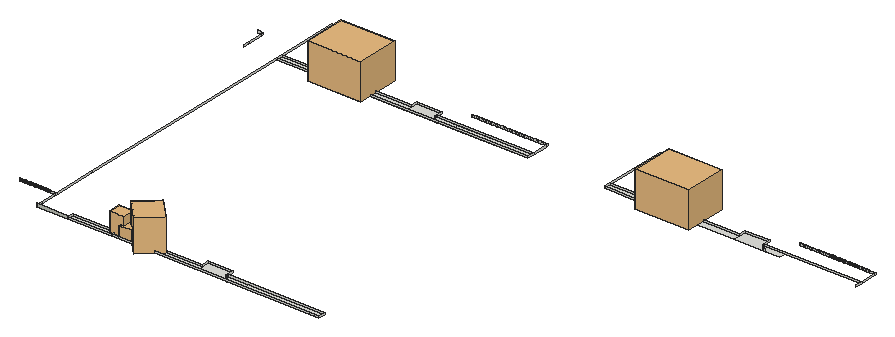
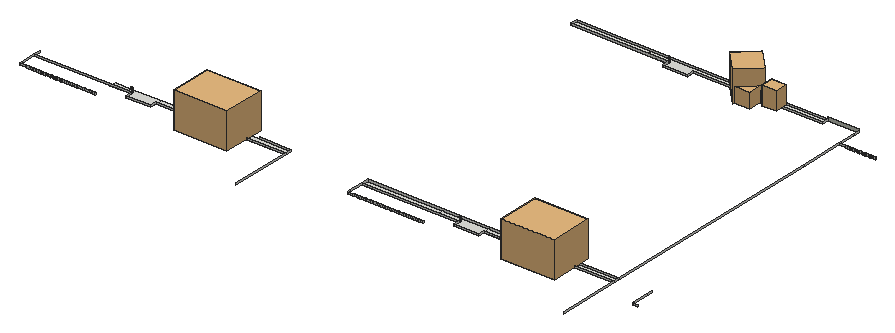
# SketchUp Ruby script. Lengths in inches.
U = 1.inch
M = Sketchup.active_model
def pt(a) = Geom::Point3d.new(a.map { |v| v * U })
def face(e, loops, mat)
  f = e.add_face(loops[0].map { |a| pt(a) })
  loops[1..].each { |l| e.add_face(l.map { |a| pt(a) }).erase! }
  f.material = f.back_material = mat if mat
  f
end
# faces: each face lists its corners as indices into pts; further lists are holes
def faces(e, pts, list, mat = nil) = list.each { |f| face(e, (f[0].is_a?(Array) ? f : [f]).map { |l| l.map { |i| pts[i] } }, mat) }
# xy, xz, yz: faces in a plane at the given z, y or x. An outline is a flat list of corners, or four numbers for a rectangle; further outlines are holes
def ring(l) = l.size == 4 ? [[l[0], l[1]], [l[2], l[1]], [l[2], l[3]], [l[0], l[3]]] : l.each_slice(2).to_a
def flat(e, list, mat, &to3) = list.each { |f| face(e, (f[0].is_a?(Array) ? f : [f]).map { |l| ring(l).map { |u, v| to3.(u, v) } }, mat) }
def xy(e, z, list, mat = nil) = flat(e, list, mat) { |x, y| [x, y, z] }
def xz(e, y, list, mat = nil) = flat(e, list, mat) { |x, z| [x, y, z] }
def yz(e, x, list, mat = nil) = flat(e, list, mat) { |y, z| [x, y, z] }
def lines(e, pts, list) = list.each { |a, b| e.add_line(pt(pts[a]), pt(pts[b])) }
# prism: a flat outline (further loops are holes) pulled along v
def prism(e, loops, v, mat = nil)
  f = face(e, loops, mat); d = Geom::Vector3d.new(v.map { |x| x * U })
  f.pushpull(f.normal.samedirection?(d) ? d.length : -d.length)
end
def box(e, o, s, mat = nil) = prism(e, [[o, [o[0] + s[0], o[1], o[2]], [o[0] + s[0], o[1] + s[1], o[2]], [o[0], o[1] + s[1], o[2]]]], [0, 0, s[2]], mat)
def at(x, y, z, deg = 0) = Geom::Transformation.translation(pt([x, y, z])) * Geom::Transformation.rotation(ORIGIN, Z_AXIS, deg.degrees)
def axes(o, x, y, z) = Geom::Transformation.new([*x, 0, *y, 0, *z, 0, *pt(o).to_a, 1])
def part(name) = M.definitions.add(name)
# library, detail: a bought-in or finely detailed component or shape, given as its bounding box
def library(name, o, s) = part(name).tap { |d| box(d.entities, o, s) }
def detail(e, o, s) = box(e.add_group.entities, o, s)
def put(e, d, t, mat = nil) = e.add_instance(d, t).tap { |i| i.material = mat if mat }
def group(e, t, mat = nil) = e.add_group.tap { |g| g.transformation = t; g.material = mat if mat }.entities
root = M.entities
M.materials.add("Material__1").color = [95, 70, 46]
M.materials.add("[Pavers with Grass Herringbone]").color = [197, 201, 190]
M.materials.add("wire_5").color = [232, 232, 232]
c1 = library("Sem+nome (1)",[20.77,3.52,-2.22],[96.42,122.82,82.56])
c2 = library("Agrupar\#178",[0,0,0],[37.88,32.09,49.42])
c3 = library("Agrupar\#177",[0,0,0],[36.52,33.08,30.88])
c4 = library("Agrupar\#154",[0,0,0],[41.26,44.6,38.97])
c5 = library("Palm",[82.2,-9.29,-2.36],[51.18,55.77,65.42])
c6 = library("Pinch Pot",[-27.95,-27.95,0],[55.9,55.9,47.42])
c7 = library("Group\#386",[-915.9375,-34.5,735.6],[41.04,40.85,6.81])
c8 = library("Group\#403",[-912.1,-32.49,735.82],[33.14,36.63,9.55])
c9 = part("Potted palm")
put(c9.entities,c5,axes([3796.42,-10488.37,43.97],[0,116.51338,0],[-116.51338,0,0],[0,0,116.51338]))
put(c9.entities,c6,axes([1647.67,1801.1875,0],[0,30.58476,0],[-30.58476,0,0],[0,0,45.1095]))
put(c9.entities,c7,axes([32580.48,2279.8125,-23417.78],[34.48768,0,0],[0,34.48768,0],[0,0,34.48768]),"Material__1")
put(c9.entities,c8,axes([32580.48,2279.8125,-23417.78],[34.48768,0,0],[0,34.48768,0],[0,0,34.48768]),"wire_5")
xy(root,-12.3125,[[1134.71,147.25,1235.9,162.52],[1300.19,147.25,1302.19,147.38,1304.14,147.77,1306.03,148.41,1307.83,149.3,1309.49,150.4,1310.99,151.72,1312.3,153.22,1313.41,154.88,1314.3,156.67,1314.9375,158.57,1315.33,160.52,1315.46,162.52,1432.9,162.52,1432.9,147.25],[1432.9,147.25,1432.9,178.0625,1489.92,178.0625,1489.92,162.33,1490.05,160.36,1490.43,158.43,1491.07,156.56,1491.9375,154.79,1493.03,153.15,1494.34,151.67,1495.82,150.37,1497.46,149.27,1499.23,148.4,1501.1,147.76,1503.03,147.38,1505,147.25],[1505,147.25,1503.03,147.38,1501.1,147.76,1499.23,148.4,1497.46,149.27,1495.82,150.37,1494.34,151.67,1493.03,153.15,1491.9375,154.79,1491.07,156.56,1490.43,158.43,1490.05,160.36,1489.92,162.33,1539,162.33,1539,147.25],[1539,147.25,1713.52,162.33],
  [1063.02,838.14,1164.21,853.41],[1228.5,838.14,1230.5,838.27,1232.46,838.66,1234.35,839.31,1236.14,840.19,1237.8,841.3,1239.3,842.62,1240.62,844.12,1241.73,845.78,1242.61,847.57,1243.25,849.46,1243.64,851.42,1243.77,853.41,1361.21,853.41,1361.21,838.14],[1361.21,838.14,1361.21,868.96,1418.23,868.96,1418.23,853.22,1418.36,851.26,1418.74,849.32,1419.38,847.45,1420.25,845.68,1421.35,844.04,1422.65,842.5625,1424.13,841.26,1425.77,840.16,1427.54,839.29,1429.41,838.66,1431.34,838.27,1433.3125,838.14],[1433.3125,838.14,1431.34,838.27,1429.41,838.66,1427.54,839.29,1425.77,840.16,1424.13,841.26,1422.65,842.5625,1421.35,844.04,1420.25,845.68,1419.38,847.45,1418.74,849.32,1418.36,851.26,1418.23,853.22,1467.3125,853.22,1467.3125,838.14],[1467.3125,838.14,1641.83,853.22],
  [1817.65,838.14,1918.83,853.41],[1983.13,838.14,1985.12,838.27,1987.08,838.66,1988.97,839.31,1990.76,840.19,1992.42,841.3,1993.93,842.62,1995.24,844.12,1996.35,845.78,1997.23,847.57,1997.875,849.46,1998.27,851.42,1998.4,853.41,2115.83,853.41,2115.83,838.14],[2115.83,838.14,2115.83,868.96,2172.86,868.96,2172.86,853.22,2172.98,851.26,2173.37,849.32,2174,847.45,2174.875,845.68,2175.97,844.04,2177.27,842.5625,2178.76,841.26,2180.4,840.16,2182.17,839.29,2184.03,838.66,2185.97,838.27,2187.9375,838.14],[2187.9375,838.14,2185.97,838.27,2184.03,838.66,2182.17,839.29,2180.4,840.16,2178.76,841.26,2177.27,842.5625,2175.97,844.04,2174.875,845.68,2174,847.45,2173.37,849.32,2172.98,851.26,2172.86,853.22,2221.9375,853.22,2221.9375,838.14]])
xz(root,147.25,[[1134.71,-12.3125,1235.9,-8],[1235.9,-12.3125,1300.19,-8],[1300.19,-12.3125,1713.52,-8]])
xz(root,147.25,[[1063.02,-12.3125,1134.71,-4.67]],"[Pavers with Grass Herringbone]")
xz(root,162.33,[[1489.92,-12.3125,1713.52,-8]])
xz(root,162.52,[[1134.71,-12.3125,1235.9,-8],[1235.9,-12.3125,1315.46,-8],[1315.46,-12.3125,1432.9,-8]])
xz(root,178.0625,[[1432.9,-12.3125,1489.92,-8]])
xz(root,203.875,[[978.875,-12.3125,982.125,-8],[982.875,-12.3125,986.125,-8],[986.875,-12.3125,990.125,-8],[990.875,-12.3125,994.125,-8],[994.875,-12.3125,998.125,-8],
  [998.875,-12.3125,1002.125,-8],[1002.875,-12.3125,1006.125,-8],[1006.875,-12.3125,1010.125,-8],[1010.875,-12.3125,1014.125,-8],[1014.875,-12.3125,1018.125,-8],
  [1018.875,-12.3125,1022.125,-8],[1022.875,-12.3125,1026.125,-8],[1026.875,-12.3125,1030.125,-8],[1030.875,-12.3125,1034.125,-8],[1034.875,-12.3125,1038.125,-8],
  [1038.875,-12.3125,1042.125,-8],[1042.875,-12.3125,1046.125,-8],[1046.875,-12.3125,1050.125,-8],[1050.125,-12.3125,1063.02,-8]])
xz(root,204.875,[[978.125,-12.3125,978.875,-8],[982.125,-12.3125,982.875,-8],[986.125,-12.3125,986.875,-8],[990.125,-12.3125,990.875,-8],[994.125,-12.3125,994.875,-8],
  [998.125,-12.3125,998.875,-8],[1002.125,-12.3125,1002.875,-8],[1006.125,-12.3125,1006.875,-8],[1010.125,-12.3125,1010.875,-8],[1014.125,-12.3125,1014.875,-8],
  [1018.125,-12.3125,1018.875,-8],[1022.125,-12.3125,1022.875,-8],[1026.125,-12.3125,1026.875,-8],[1030.125,-12.3125,1030.875,-8],[1034.125,-12.3125,1034.875,-8],
  [1038.125,-12.3125,1038.875,-8],[1042.125,-12.3125,1042.875,-8],[1046.125,-12.3125,1046.875,-8]])
xz(root,838.14,[[1063.02,-12.3125,1134.71,-8],[1134.71,-12.3125,1164.21,-8],[1164.21,-12.3125,1228.5,-8],[1228.5,-12.3125,1641.83,-8],[1817.65,-12.3125,1889.33,-8],
  [1918.83,-12.3125,1983.13,-8]])
xz(root,853.22,[[1418.23,-12.3125,1641.83,-8],[2172.86,-12.3125,2396.46,-8]])
xz(root,853.41,[[1063.02,-12.3125,1164.21,-8],[1164.21,-12.3125,1243.77,-8],[1243.77,-12.3125,1361.21,-8],[1817.65,-12.3125,1918.83,-8],[1918.83,-12.3125,1998.4,-8],
  [1998.4,-12.3125,2115.83,-8]])
xz(root,868.96,[[1361.21,-12.3125,1418.23,-8],[2115.83,-12.3125,2172.86,-8]])
xz(root,894.77,[[973.4375,-12.3125,986.33,-8],[1467.3125,-12.3125,1468.9375,-8],[1469.6875,-12.3125,1472.9375,-8],[1473.6875,-12.3125,1476.9375,-8],[1477.6875,-12.3125,1480.9375,-8],
  [1481.6875,-12.3125,1484.9375,-8],[1485.6875,-12.3125,1488.9375,-8],[1489.6875,-12.3125,1492.9375,-8],[1493.6875,-12.3125,1496.9375,-8],[1497.6875,-12.3125,1500.9375,-8],
  [1501.6875,-12.3125,1504.9375,-8],[1505.6875,-12.3125,1508.9375,-8],[1509.6875,-12.3125,1512.9375,-8],[1513.6875,-12.3125,1516.9375,-8],[1517.6875,-12.3125,1520.9375,-8],
  [1521.6875,-12.3125,1524.9375,-8],[1525.6875,-12.3125,1528.9375,-8],[1529.6875,-12.3125,1532.9375,-8],[1533.6875,-12.3125,1536.9375,-8],[1537.6875,-12.3125,1540.9375,-8],
  [1541.6875,-12.3125,1544.9375,-8],[1545.6875,-12.3125,1548.9375,-8],[1549.6875,-12.3125,1552.9375,-8],[1553.6875,-12.3125,1556.9375,-8],[1557.6875,-12.3125,1560.9375,-8],
  [1561.6875,-12.3125,1564.9375,-8],[1565.6875,-12.3125,1568.9375,-8],[1569.6875,-12.3125,1572.9375,-8],[1573.6875,-12.3125,1576.9375,-8],[1577.6875,-12.3125,1580.9375,-8],
  [1581.6875,-12.3125,1584.9375,-8],[1585.6875,-12.3125,1588.9375,-8],[1589.6875,-12.3125,1592.9375,-8],[1593.6875,-12.3125,1596.9375,-8],[1597.6875,-12.3125,1600.9375,-8],
  [1601.6875,-12.3125,1604.9375,-8],[1605.6875,-12.3125,1608.9375,-8],[1609.6875,-12.3125,1612.9375,-8],[1613.6875,-12.3125,1616.9375,-8],[1617.6875,-12.3125,1620.9375,-8],
  [1621.6875,-12.3125,1624.9375,-8],[1625.6875,-12.3125,1628.9375,-8],[1628.9375,-12.3125,1641.83,-8],[2221.9375,-12.3125,2223.5625,-8],[2224.3125,-12.3125,2227.5625,-8],
  [2228.3125,-12.3125,2231.5625,-8],[2232.3125,-12.3125,2235.5625,-8],[2236.3125,-12.3125,2239.5625,-8],[2240.3125,-12.3125,2243.5625,-8],[2244.3125,-12.3125,2247.5625,-8],
  [2248.3125,-12.3125,2251.5625,-8],[2252.3125,-12.3125,2255.5625,-8],[2256.3125,-12.3125,2259.5625,-8],[2260.3125,-12.3125,2263.5625,-8],[2264.3125,-12.3125,2267.5625,-8],
  [2268.3125,-12.3125,2271.5625,-8],[2272.3125,-12.3125,2275.5625,-8],[2276.3125,-12.3125,2279.5625,-8],[2280.3125,-12.3125,2283.5625,-8],[2284.3125,-12.3125,2287.5625,-8],
  [2288.3125,-12.3125,2291.5625,-8],[2292.3125,-12.3125,2295.5625,-8],[2296.3125,-12.3125,2299.5625,-8],[2300.3125,-12.3125,2303.5625,-8],[2304.3125,-12.3125,2307.5625,-8],
  [2308.3125,-12.3125,2311.5625,-8],[2312.3125,-12.3125,2315.5625,-8],[2316.3125,-12.3125,2319.5625,-8],[2320.3125,-12.3125,2323.5625,-8],[2324.3125,-12.3125,2327.5625,-8],
  [2328.3125,-12.3125,2331.5625,-8],[2332.3125,-12.3125,2335.5625,-8],[2336.3125,-12.3125,2339.5625,-8],[2340.3125,-12.3125,2343.5625,-8],[2344.3125,-12.3125,2347.5625,-8],
  [2348.3125,-12.3125,2351.5625,-8],[2352.3125,-12.3125,2355.5625,-8],[2356.3125,-12.3125,2359.5625,-8],[2360.3125,-12.3125,2363.5625,-8],[2364.3125,-12.3125,2367.5625,-8],
  [2368.3125,-12.3125,2371.5625,-8],[2372.3125,-12.3125,2375.5625,-8],[2376.3125,-12.3125,2379.5625,-8],[2380.3125,-12.3125,2383.5625,-8],[2383.5625,-12.3125,2396.46,-8]])
xz(root,895.77,[[2291.5625,-12.3125,2292.3125,-8],[2295.5625,-12.3125,2296.3125,-8],[2307.5625,-12.3125,2308.3125,-8],[2311.5625,-12.3125,2312.3125,-8],[2315.5625,-12.3125,2316.3125,-8],
  [2323.5625,-12.3125,2324.3125,-8],[2331.5625,-12.3125,2332.3125,-8],[2335.5625,-12.3125,2336.3125,-8],[2339.5625,-12.3125,2340.3125,-8],[2343.5625,-12.3125,2344.3125,-8],
  [2347.5625,-12.3125,2348.3125,-8],[2351.5625,-12.3125,2352.3125,-8],[2355.5625,-12.3125,2356.3125,-8]])
yz(root,978.875,[[203.875,-12.3125,204.875,-8]])
yz(root,982.125,[[203.875,-12.3125,204.875,-8]])
yz(root,982.875,[[203.875,-12.3125,204.875,-8]])
yz(root,986.125,[[203.875,-12.3125,204.875,-8]])
yz(root,986.33,[[838.14,-12.3125,853.22,-8],[853.22,-12.3125,889.52,-8],[889.52,-12.3125,894.77,-8]])
yz(root,986.875,[[203.875,-12.3125,204.875,-8]])
yz(root,990.125,[[203.875,-12.3125,204.875,-8]])
yz(root,990.875,[[203.875,-12.3125,204.875,-8]])
yz(root,994.125,[[203.875,-12.3125,204.875,-8]])
yz(root,994.875,[[203.875,-12.3125,204.875,-8]])
yz(root,998.125,[[203.875,-12.3125,204.875,-8]])
yz(root,998.875,[[203.875,-12.3125,204.875,-8]])
yz(root,1002.125,[[203.875,-12.3125,204.875,-8]])
yz(root,1002.875,[[203.875,-12.3125,204.875,-8]])
yz(root,1006.125,[[203.875,-12.3125,204.875,-8]])
yz(root,1006.875,[[203.875,-12.3125,204.875,-8]])
yz(root,1010.125,[[203.875,-12.3125,204.875,-8]])
yz(root,1010.875,[[203.875,-12.3125,204.875,-8]])
yz(root,1014.125,[[203.875,-12.3125,204.875,-8]])
yz(root,1014.875,[[203.875,-12.3125,204.875,-8]])
yz(root,1018.125,[[203.875,-12.3125,204.875,-8]])
yz(root,1018.875,[[203.875,-12.3125,204.875,-8]])
yz(root,1022.125,[[203.875,-12.3125,204.875,-8]])
yz(root,1022.875,[[203.875,-12.3125,204.875,-8]])
yz(root,1026.125,[[203.875,-12.3125,204.875,-8]])
yz(root,1026.875,[[203.875,-12.3125,204.875,-8]])
yz(root,1030.125,[[203.875,-12.3125,204.875,-8]])
yz(root,1030.875,[[203.875,-12.3125,204.875,-8]])
yz(root,1034.125,[[203.875,-12.3125,204.875,-8]])
yz(root,1034.875,[[203.875,-12.3125,204.875,-8]])
yz(root,1038.125,[[203.875,-12.3125,204.875,-8]])
yz(root,1038.875,[[203.875,-12.3125,204.875,-8]])
yz(root,1042.125,[[203.875,-12.3125,204.875,-8]])
yz(root,1042.875,[[203.875,-12.3125,204.875,-8]])
yz(root,1046.125,[[203.875,-12.3125,204.875,-8]])
yz(root,1046.875,[[203.875,-12.3125,204.875,-8]])
yz(root,1063.02,[[147.25,-12.3125,162.33,-8],[162.33,-12.3125,198.625,-8],[198.625,-12.3125,203.875,-8],[203.875,-12.3125,305.58,-8],[305.58,-12.3125,838.14,-8],
  [838.14,-12.3125,853.41,-8],[853.41,-12.3125,996.48,-8]])
yz(root,1134.71,[[147.25,-12.3125,162.52,-8]])
yz(root,1164.21,[[838.14,-12.3125,853.41,-8]])
yz(root,1235.9,[[147.25,-12.3125,162.52,-8]])
yz(root,1361.21,[[853.41,-12.3125,868.96,-8]])
yz(root,1418.23,[[853.22,-12.3125,868.96,-8]])
yz(root,1432.9,[[162.52,-12.3125,178.0625,-8]])
yz(root,1489.92,[[162.33,-12.3125,178.0625,-8]])
yz(root,1641.83,[[838.14,-12.3125,853.22,-8],[853.22,-12.3125,889.52,-8],[889.52,-12.3125,894.77,-8]])
yz(root,1713.52,[[147.25,-12.3125,162.33,-8]])
yz(root,1817.65,[[838.14,-12.3125,853.41,-8],[853.41,-12.3125,996.48,-8]])
yz(root,1918.83,[[838.14,-12.3125,853.41,-8]])
yz(root,2115.83,[[853.41,-12.3125,868.96,-8]])
yz(root,2172.86,[[853.22,-12.3125,868.96,-8]])
yz(root,2268.3125,[[894.77,-12.3125,895.77,-8]])
yz(root,2291.5625,[[894.77,-12.3125,895.77,-8]])
yz(root,2295.5625,[[894.77,-12.3125,895.77,-8]])
yz(root,2296.3125,[[894.77,-12.3125,895.77,-8]])
yz(root,2299.5625,[[894.77,-12.3125,895.77,-8]])
yz(root,2300.3125,[[894.77,-12.3125,895.77,-8]])
yz(root,2307.5625,[[894.77,-12.3125,895.77,-8]])
yz(root,2308.3125,[[894.77,-12.3125,895.77,-8]])
yz(root,2311.5625,[[894.77,-12.3125,895.77,-8]])
yz(root,2312.3125,[[894.77,-12.3125,895.77,-8]])
yz(root,2316.3125,[[894.77,-12.3125,895.77,-8]])
yz(root,2319.5625,[[894.77,-12.3125,895.77,-8]])
yz(root,2324.3125,[[894.77,-12.3125,895.77,-8]])
yz(root,2332.3125,[[894.77,-12.3125,895.77,-8]])
yz(root,2336.3125,[[894.77,-12.3125,895.77,-8]])
yz(root,2339.5625,[[894.77,-12.3125,895.77,-8]])
yz(root,2344.3125,[[894.77,-12.3125,895.77,-8]])
yz(root,2347.5625,[[894.77,-12.3125,895.77,-8]])
yz(root,2348.3125,[[894.77,-12.3125,895.77,-8]])
yz(root,2351.5625,[[894.77,-12.3125,895.77,-8]])
yz(root,2352.3125,[[894.77,-12.3125,895.77,-8]])
yz(root,2355.5625,[[894.77,-12.3125,895.77,-8]])
yz(root,2396.46,[[838.14,-12.3125,853.22,-8],[853.22,-12.3125,889.52,-8],[889.52,-12.3125,894.77,-8]])
p = [[1302.19,147.38,-8],[1300.19,147.25,-8],[1300.19,147.25,-12.3125],[1302.19,147.38,-12.3125],[1304.14,147.77,-8],[1304.14,147.77,-12.3125],
  [1503.03,147.38,-8],[1501.1,147.76,-8],[1501.1,147.76,-12.3125],[1503.03,147.38,-12.3125],[1306.03,148.41,-8],[1306.03,148.41,-12.3125],
  [1499.23,148.4,-8],[1499.23,148.4,-12.3125],[1307.83,149.3,-8],[1307.83,149.3,-12.3125],[1497.46,149.27,-8],[1497.46,149.27,-12.3125],
  [1309.49,150.4,-8],[1309.49,150.4,-12.3125],[1495.82,150.37,-8],[1495.82,150.37,-12.3125],[1310.99,151.72,-8],[1310.99,151.72,-12.3125],
  [1494.34,151.67,-8],[1494.34,151.67,-12.3125],[1312.3,153.22,-8],[1312.3,153.22,-12.3125],[1493.03,153.15,-8],[1493.03,153.15,-12.3125],
  [1313.41,154.88,-8],[1313.41,154.88,-12.3125],[1491.9375,154.79,-8],[1491.9375,154.79,-12.3125],[1491.07,156.56,-8],[1491.07,156.56,-12.3125],
  [1314.3,156.67,-8],[1314.3,156.67,-12.3125],[1490.43,158.43,-8],[1490.43,158.43,-12.3125],[1314.9375,158.57,-8],[1314.9375,158.57,-12.3125],
  [1490.05,160.36,-8],[1490.05,160.36,-12.3125],[1315.33,160.52,-8],[1315.33,160.52,-12.3125],[1489.92,162.33,-8],[1489.92,162.33,-12.3125],
  [1315.46,162.52,-8],[1315.46,162.52,-12.3125],[1230.5,838.27,-8],[1228.5,838.14,-8],[1228.5,838.14,-12.3125],[1230.5,838.27,-12.3125],
  [1985.12,838.27,-8],[1983.13,838.14,-8],[1983.13,838.14,-12.3125],[1985.12,838.27,-12.3125],[1232.46,838.66,-8],[1232.46,838.66,-12.3125],
  [1431.34,838.27,-8],[1429.41,838.66,-8],[1429.41,838.66,-12.3125],[1431.34,838.27,-12.3125],[1987.08,838.66,-8],[1987.08,838.66,-12.3125],
  [2185.97,838.27,-8],[2184.03,838.66,-8],[2184.03,838.66,-12.3125],[2185.97,838.27,-12.3125],[1234.35,839.31,-8],[1234.35,839.31,-12.3125],
  [1427.54,839.29,-8],[1427.54,839.29,-12.3125],[1988.97,839.31,-8],[1988.97,839.31,-12.3125],[2182.17,839.29,-8],[2182.17,839.29,-12.3125],
  [1236.14,840.19,-8],[1236.14,840.19,-12.3125],[1425.77,840.16,-8],[1425.77,840.16,-12.3125],[1990.76,840.19,-8],[1990.76,840.19,-12.3125],
  [2180.4,840.16,-8],[2180.4,840.16,-12.3125],[1237.8,841.3,-8],[1237.8,841.3,-12.3125],[1424.13,841.26,-8],[1424.13,841.26,-12.3125],
  [1992.42,841.3,-8],[1992.42,841.3,-12.3125],[2178.76,841.26,-8],[2178.76,841.26,-12.3125],[1239.3,842.62,-8],[1239.3,842.62,-12.3125],
  [1422.65,842.5625,-8],[1422.65,842.5625,-12.3125],[1993.93,842.62,-8],[1993.93,842.62,-12.3125],[2177.27,842.5625,-8],[2177.27,842.5625,-12.3125],
  [1240.62,844.12,-8],[1240.62,844.12,-12.3125],[1421.35,844.04,-8],[1421.35,844.04,-12.3125],[1995.24,844.12,-8],[1995.24,844.12,-12.3125],
  [2175.97,844.04,-8],[2175.97,844.04,-12.3125],[1420.25,845.68,-8],[1420.25,845.68,-12.3125],[2174.875,845.68,-8],[2174.875,845.68,-12.3125],
  [1241.73,845.78,-8],[1241.73,845.78,-12.3125],[1996.35,845.78,-8],[1996.35,845.78,-12.3125],[1419.38,847.45,-8],[1419.38,847.45,-12.3125],
  [2174,847.45,-8],[2174,847.45,-12.3125],[1242.61,847.57,-8],[1242.61,847.57,-12.3125],[1997.23,847.57,-8],[1997.23,847.57,-12.3125],
  [1418.74,849.32,-8],[1418.74,849.32,-12.3125],[2173.37,849.32,-8],[2173.37,849.32,-12.3125],[1243.25,849.46,-8],[1243.25,849.46,-12.3125],
  [1997.875,849.46,-8],[1997.875,849.46,-12.3125],[1418.36,851.26,-8],[1418.36,851.26,-12.3125],[2172.98,851.26,-8],[2172.98,851.26,-12.3125],
  [1243.64,851.42,-8],[1243.64,851.42,-12.3125],[1998.27,851.42,-8],[1998.27,851.42,-12.3125],[1418.23,853.22,-8],[1418.23,853.22,-12.3125],
  [2172.86,853.22,-8],[2172.86,853.22,-12.3125],[1243.77,853.41,-8],[1243.77,853.41,-12.3125],[1998.4,853.41,-8],[1998.4,853.41,-12.3125],
  [1263.22,209.33,-9.96],[1262.8,208.91,-9.96],[1263.22,208.91,-9.96]]
faces(root,p,[[0,1,2,3],[4,0,3,5],[6,7,8,9],[10,4,5,11],[7,12,13,8],[14,10,11,15],[12,16,17,13],[18,14,15,19],
  [16,20,21,17],[22,18,19,23],[20,24,25,21],[26,22,23,27],[24,28,29,25],[30,26,27,31],[28,32,33,29],[32,34,35,33],
  [36,30,31,37],[34,38,39,35],[40,36,37,41],[38,42,43,39],[44,40,41,45],[42,46,47,43],[48,44,45,49],[50,51,52,53],
  [54,55,56,57],[58,50,53,59],[60,61,62,63],[64,54,57,65],[66,67,68,69],[70,58,59,71],[61,72,73,62],[74,64,65,75],
  [67,76,77,68],[78,70,71,79],[72,80,81,73],[82,74,75,83],[76,84,85,77],[86,78,79,87],[80,88,89,81],[90,82,83,91],
  [84,92,93,85],[94,86,87,95],[88,96,97,89],[98,90,91,99],[92,100,101,93],[102,94,95,103],[96,104,105,97],[106,98,99,107],
  [100,108,109,101],[104,110,111,105],[108,112,113,109],[114,102,103,115],[116,106,107,117],[110,118,119,111],[112,120,121,113],[122,114,115,123],
  [124,116,117,125],[118,126,127,119],[120,128,129,121],[130,122,123,131],[132,124,125,133],[126,134,135,127],[128,136,137,129],[138,130,131,139],
  [140,132,133,141],[134,142,143,135],[136,144,145,137],[146,138,139,147],[148,140,141,149]])
lines(root,p,[[150,151],[151,152],[152,150]])
put(root,c1,at(1150.29,929.97,-10.09,-90))
put(root,c2,axes([1225.5,153.88,-9.51],[0.87,0,0],[0,0.87,0],[0,0,0.87]))
put(root,c3,axes([1251.78,148.8,-9.3],[0.79,0,0],[0,0.79,0],[0,0,0.79]))
put(root,c4,axes([1268.42,166.15,-10.09],[0.89,0,0],[0,0.89,0],[0,0,0.89]))
put(root,c9,axes([1309.75,189.25,-10.09],[0.0066,-0.00697,0],[-0.00697,-0.0066,0],[0,0,0.0096]))
put(root,c1,at(1904.92,929.97,-10.09,-90))
